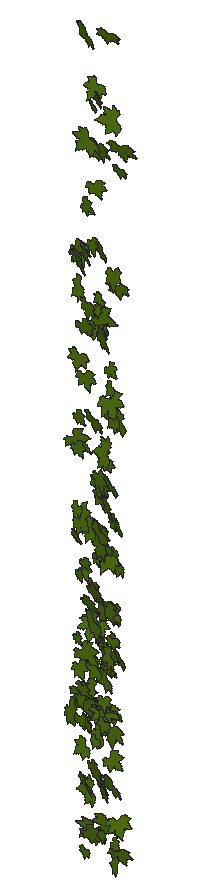
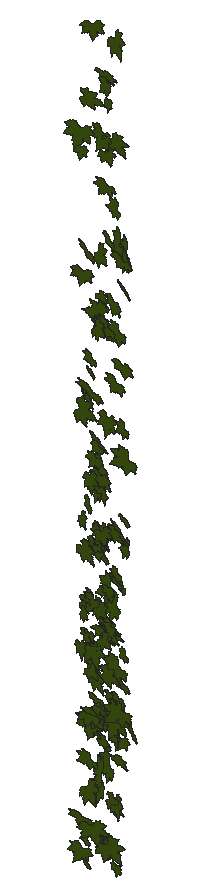
# SketchUp Ruby script. Lengths in inches.
U = 1.inch
M = Sketchup.active_model
def pt(a) = Geom::Point3d.new(a.map { |v| v * U })
def face(e, loops, mat)
  f = e.add_face(loops[0].map { |a| pt(a) })
  loops[1..].each { |l| e.add_face(l.map { |a| pt(a) }).erase! }
  f.material = f.back_material = mat if mat
  f
end
# faces: each face lists its corners as indices into pts; further lists are holes
def faces(e, pts, list, mat = nil) = list.each { |f| face(e, (f[0].is_a?(Array) ? f : [f]).map { |l| l.map { |i| pts[i] } }, mat) }
# xy, xz, yz: faces in a plane at the given z, y or x. An outline is a flat list of corners, or four numbers for a rectangle; further outlines are holes
def ring(l) = l.size == 4 ? [[l[0], l[1]], [l[2], l[1]], [l[2], l[3]], [l[0], l[3]]] : l.each_slice(2).to_a
def flat(e, list, mat, &to3) = list.each { |f| face(e, (f[0].is_a?(Array) ? f : [f]).map { |l| ring(l).map { |u, v| to3.(u, v) } }, mat) }
def xy(e, z, list, mat = nil) = flat(e, list, mat) { |x, y| [x, y, z] }
def xz(e, y, list, mat = nil) = flat(e, list, mat) { |x, z| [x, y, z] }
def yz(e, x, list, mat = nil) = flat(e, list, mat) { |y, z| [x, y, z] }
def lines(e, pts, list) = list.each { |a, b| e.add_line(pt(pts[a]), pt(pts[b])) }
# prism: a flat outline (further loops are holes) pulled along v
def prism(e, loops, v, mat = nil)
  f = face(e, loops, mat); d = Geom::Vector3d.new(v.map { |x| x * U })
  f.pushpull(f.normal.samedirection?(d) ? d.length : -d.length)
end
def box(e, o, s, mat = nil) = prism(e, [[o, [o[0] + s[0], o[1], o[2]], [o[0] + s[0], o[1] + s[1], o[2]], [o[0], o[1] + s[1], o[2]]]], [0, 0, s[2]], mat)
def at(x, y, z, deg = 0) = Geom::Transformation.translation(pt([x, y, z])) * Geom::Transformation.rotation(ORIGIN, Z_AXIS, deg.degrees)
def axes(o, x, y, z) = Geom::Transformation.new([*x, 0, *y, 0, *z, 0, *pt(o).to_a, 1])
def part(name) = M.definitions.add(name)
# library, detail: a bought-in or finely detailed component or shape, given as its bounding box
def library(name, o, s) = part(name).tap { |d| box(d.entities, o, s) }
def detail(e, o, s) = box(e.add_group.entities, o, s)
def put(e, d, t, mat = nil) = e.add_instance(d, t).tap { |i| i.material = mat if mat }
def group(e, t, mat = nil) = e.add_group.tap { |g| g.transformation = t; g.material = mat if mat }.entities
root = M.entities
M.materials.add("[Vegetation Blur 03]").color = [83, 114, 18]
c1 = part("ivy")
xy(c1.entities,0,[[0.782,0,0.786,0,0.787,0.005,0.789,0.009,0.821,0.072,0.875,0.147,1.001,0.272,1.073,0.331,1.137,0.363,1.178,0.379,1.223,0.384,1.272,0.383,1.311,0.374,1.36,0.355,1.399,0.334,1.491,0.285,1.541,0.244,1.583,0.199,1.617,0.15,1.64,0.128,1.662,0.115,1.717,0.105,1.745,0.093,1.784,0.054,1.819,0.057,1.854,0.064,1.882,0.075,1.896,0.074,1.91,0.071,1.937,0.063,1.964,0.053,1.99,0.038,2.016,0.015,2.034,0.002,2.04,0,2.038,0.003,2.036,0.007,2.033,0.038,2.036,0.068,2.045,0.1,2.055,0.116,2.064,0.123,2.077,0.129,2.088,0.129,2.106,0.132,2.118,0.13,2.179,0.132,2.207,0.133,2.225,0.133,2.242,0.138,2.22,0.162,2.207,0.186,2.206,0.213,2.212,0.236,2.228,0.262,2.247,0.274,2.298,0.283,2.355,0.294,2.37,0.296,2.376,0.295,2.377,0.3,2.377,0.303,2.385,0.329,2.411,0.37,2.426,0.392,2.449,0.407,2.511,0.426,2.561,0.444,2.619,0.466,2.589,0.469,2.561,0.476,2.501,0.5,2.449,0.516,2.424,0.523,2.401,0.535,2.377,0.556,2.372,0.568,2.36,0.575,2.268,0.586,2.225,0.592,2.207,0.599,2.194,0.61,2.143,0.65,2.13,0.664,2.122,0.682,2.123,0.7,2.13,0.719,2.148,0.75,2.17,0.781,2.195,0.807,2.221,0.828,2.284,0.874,2.291,0.88,2.288,0.887,2.276,0.9,2.267,0.916,2.265,0.933,2.273,0.967,2.292,1.002,2.313,1.03,2.334,1.054,2.348,1.067,2.358,1.074,2.363,1.076,2.362,1.081,2.35,1.094,2.347,1.11,2.35,1.143,2.359,1.18,2.385,1.254,2.415,1.324,2.448,1.393,2.45,1.4,2.446,1.398,2.44,1.394,2.427,1.383,2.402,1.36,2.376,1.339,2.345,1.324,2.305,1.309,2.282,1.303,2.273,1.306,2.245,1.294,2.212,1.287,2.187,1.291,2.163,1.301,2.142,1.316,2.134,1.327,2.124,1.325,2.09,1.292,2.053,1.259,2.014,1.234,1.973,1.215,1.954,1.21,1.931,1.208,1.909,1.212,1.893,1.22,1.879,1.233,1.872,1.248,1.867,1.281,1.864,1.319,1.821,1.258,1.773,1.197,1.726,1.141,1.698,1.121,1.679,1.116,1.666,1.117,1.647,1.122,1.632,1.129,1.62,1.141,1.617,1.154,1.617,1.219,1.621,1.254,1.623,1.268,1.623,1.281,1.618,1.314,1.606,1.346,1.603,1.375,1.607,1.403,1.603,1.467,1.599,1.499,1.605,1.525,1.614,1.552,1.629,1.577,1.635,1.589,1.629,1.587,1.618,1.582,1.596,1.566,1.581,1.556,1.568,1.552,1.557,1.55,1.545,1.553,1.531,1.562,1.522,1.572,1.504,1.591,1.486,1.611,1.474,1.631,1.457,1.666,1.455,1.684,1.457,1.698,1.452,1.715,1.444,1.728,1.424,1.754,1.419,1.772,1.423,1.786,1.434,1.819,1.444,1.848,1.446,1.855,1.44,1.861,1.43,1.867,1.386,1.904,1.349,1.948,1.326,1.973,1.31,1.995,1.288,2.048,1.284,2.153,1.287,2.254,1.284,2.255,1.282,2.253,1.278,2.247,1.274,2.237,1.266,2.216,1.226,2.125,1.208,2.076,1.184,2.033,1.155,1.984,1.135,1.942,1.111,1.899,1.083,1.861,1.053,1.85,1.059,1.83,1.061,1.809,1.056,1.79,1.049,1.767,1.04,1.749,1.018,1.733,0.994,1.726,0.942,1.734,0.95,1.6875,0.944,1.645,0.932,1.608,0.911,1.585,0.881,1.58,0.854,1.582,0.828,1.588,0.785,1.618,0.773,1.625,0.775,1.614,0.779,1.598,0.796,1.502,0.818,1.402,0.861,1.283,0.882,1.224,0.894,1.174,0.892,1.148,0.886,1.123,0.881,1.107,0.872,1.099,0.849,1.094,0.818,1.092,0.789,1.098,0.762,1.107,0.753,1.113,0.721,1.139,0.698,1.163,0.678,1.194,0.665,1.224,0.628,1.28,0.612,1.312,0.606,1.327,0.606,1.314,0.599,1.282,0.594,1.267,0.581,1.256,0.544,1.245,0.512,1.244,0.473,1.249,0.444,1.256,0.382,1.288,0.339,1.306,0.324,1.316,0.317,1.324,0.309,1.326,0.27,1.314,0.227,1.313,0.185,1.3125,0.152,1.317,0.122,1.328,0.092,1.345,0.073,1.353,0.079,1.338,0.092,1.308,0.117,1.249,0.13,1.215,0.139,1.164,0.147,1.148,0.157,1.136,0.163,1.122,0.174,1.086,0.177,1.067,0.182,1.054,0.186,1.043,0.191,1.038,0.211,1.028,0.237,1.005,0.25,0.974,0.253,0.96,0.25,0.944,0.242,0.914,0.243,0.906,0.249,0.902,0.26,0.894,0.289,0.88,0.307,0.873,0.322,0.862,0.364,0.799,0.403,0.738,0.431,0.709,0.439,0.691,0.441,0.678,0.4375,0.66,0.428,0.645,0.394,0.623,0.303,0.594,0.255,0.581,0.214,0.577,0.179,0.573,0.173,0.568,0.175,0.561,0.167,0.55,0.141,0.523,0.113,0.503,0.077,0.49,0.045,0.486,0.026,0.485,0.019,0.486,0.011,0.483,0,0.471,0.014,0.467,0.044,0.455,0.058,0.447,0.07,0.438,0.097,0.411,0.125,0.394,0.158,0.377,0.174,0.366,0.182,0.359,0.185,0.361,0.242,0.331,0.253,0.316,0.258,0.303,0.262,0.283,0.274,0.278,0.308,0.274,0.341,0.252,0.366,0.226,0.366,0.222,0.37,0.22,0.38,0.221,0.395,0.221,0.425,0.216,0.45,0.207,0.465,0.192,0.473,0.178,0.484,0.15,0.489,0.116,0.483,0.089,0.468,0.058,0.45,0.035,0.435,0.018,0.429,0.011,0.434,0.012,0.438,0.014,0.469,0.019,0.542,0.016,0.581,0.015,0.612,0.027,0.68,0.055,0.696,0.057,0.712,0.052,0.73,0.045,0.741,0.036,0.766,0.014]])
put(root,c1,axes([74.63,173.7,60.75],[0.26152,-0.04302,0.44662],[0.5117,-0.42542,-0.20602],[-0.19512,-1.17335,0.05832]),"[Vegetation Blur 03]")
put(root,c1,axes([74.51,173.7,74.86],[0.3615,0.01419,0.44771],[0.54841,0.02846,-0.29509],[0.01534,-1.35164,-0.00151]),"[Vegetation Blur 03]")
put(root,c1,axes([75.65,173.7,97.39],[0.37946,-0.0754,-0.40939],[-0.47883,0.34147,-0.30552],[-0.15388,-1.24846,-0.05884]),"[Vegetation Blur 03]")
put(root,c1,axes([75.28,173.7,72.12],[0.34373,-0.18323,-0.04475],[-0.06771,-0.09451,-0.28552],[-0.07969,-0.71,0.04955]),"[Vegetation Blur 03]")
put(root,c1,axes([75.15,173.7,64.84],[0.19414,-0.08015,0.20136],[0.24242,-0.09451,-0.1616],[-0.0602,-0.6391,-0.00136]),"[Vegetation Blur 03]")
put(root,c1,axes([75.01,173.7,80.1],[0.54066,-0.11979,-0.01485],[-0.02304,-0.09186,-0.44216],[-0.05647,-1.10941,0.03821]),"[Vegetation Blur 03]")
put(root,c1,axes([74.99,173.7,74.84],[0.30004,-0.03578,0.23182],[0.28092,-0.09842,-0.24458],[-0.04545,-0.84451,0.01868]),"[Vegetation Blur 03]")
put(root,c1,axes([75.03,173.7,60.78],[0.44477,-0.01678,0.0841],[0.10333,0.04659,-0.36253],[-0.00282,-0.93833,-0.0195]),"[Vegetation Blur 03]")
put(root,c1,axes([75.14,173.7,70.17],[0.15681,-0.19135,0.27864],[0.34217,-0.11382,-0.14055],[-0.09017,-0.7647,-0.0488]),"[Vegetation Blur 03]")
put(root,c1,axes([75.1,173.7,76.4375],[0.23733,-0.08095,0.26556],[0.32364,-0.07275,-0.19614],[-0.05179,-0.82556,-0.00876]),"[Vegetation Blur 03]")
put(root,c1,axes([74.89,173.7,85.21],[0.44354,0.00148,0.25414],[0.30752,-0.17731,-0.35733],[-0.04893,-1.101,0.05789]),"[Vegetation Blur 03]")
put(root,c1,axes([75.64,173.7,57.88],[0.41747,-0.18159,-0.28175],[-0.32214,0.27535,-0.34584],[-0.15229,-1.08022,-0.04079]),"[Vegetation Blur 03]")
put(root,c1,axes([75.3125,173.7,68.32],[0.21446,-0.11197,0.17329],[0.20462,-0.11686,-0.18055],[-0.07858,-0.60992,0.00278]),"[Vegetation Blur 03]")
put(root,c1,axes([74.93,173.7,85.11],[0.28904,-0.06987,0.39444],[0.46239,-0.30604,-0.23421],[-0.14468,-1.11768,0.03947]),"[Vegetation Blur 03]")
put(root,c1,axes([75.56,173.7,84.16],[0.42016,-0.3703,-0.17602],[-0.23818,-0.04638,-0.36333],[-0.14889,-0.97076,0.0845]),"[Vegetation Blur 03]")
put(root,c1,axes([74.8,173.7,61.94],[0.46309,-0.00814,0.32802],[0.3991,0.15897,-0.37467],[0.04767,-1.25175,-0.04972]),"[Vegetation Blur 03]")
put(root,c1,axes([75.05,173.7,63.31],[0.35031,-0.0224,0.27157],[0.32357,-0.21117,-0.28075],[-0.0784,-0.97156,0.05476]),"[Vegetation Blur 03]")
put(root,c1,axes([75.76,173.7,59.9],[0.35443,-0.19304,-0.2419],[-0.30587,-0.0509,-0.29211],[-0.05567,-0.94941,0.06485]),"[Vegetation Blur 03]")
put(root,c1,axes([75.72,173.7,91.99],[0.532,-0.08529,-0.32199],[-0.3962,-0.04622,-0.4341],[-0.01987,-1.36215,0.03489]),"[Vegetation Blur 03]")
put(root,c1,axes([75.07,173.7,70.68],[0.16553,0.17765,0.51158],[0.60894,-0.40708,-0.109],[-0.17196,-1.2705,0.10646]),"[Vegetation Blur 03]")
put(root,c1,axes([75.84,173.7,61.0625],[0.30175,-0.15566,-0.18852],[-0.22184,0.13329,-0.25383],[-0.09933,-0.77056,-0.00582]),"[Vegetation Blur 03]")
put(root,c1,axes([75.36,173.7,61.79],[0.24227,-0.06001,0.24324],[0.27574,-0.26297,-0.19314],[-0.11679,-0.74533,0.04856]),"[Vegetation Blur 03]")
put(root,c1,axes([76.33,173.7,57.9],[0.23881,-0.20013,-0.4704],[-0.57401,0.16163,-0.20491],[-0.11037,-1.27363,0.04791]),"[Vegetation Blur 03]")
put(root,c1,axes([75.59,173.7,54.07],[0.31854,-0.11206,-0.01065],[-0.01233,0.01101,-0.26373],[-0.05462,-0.65595,-0.00261]),"[Vegetation Blur 03]")
put(root,c1,axes([75.03,173.7,61.81],[0.67064,-0.03297,0.06761],[0.08405,0.14038,-0.54453],[-0.00745,-1.38343,-0.05687]),"[Vegetation Blur 03]")
put(root,c1,axes([75.37,173.7,62.65],[0.43055,-0.17357,0.04955],[0.0586,-0.03425,-0.35804],[-0.08583,-0.8941,0.0041]),"[Vegetation Blur 03]")
put(root,c1,axes([75.95,173.7,55.68],[0.46314,0.05825,-0.39602],[-0.48604,0.04033,-0.37767],[0.00535,-1.37976,-0.02776]),"[Vegetation Blur 03]")
put(root,c1,axes([75.51,173.7,68.93],[0.24085,-0.07286,0.19486],[0.23769,-0.04913,-0.19858],[-0.04198,-0.69616,-0.00638]),"[Vegetation Blur 03]")
put(root,c1,axes([76.24,173.7,71.6875],[0.31165,-0.23246,-0.38206],[-0.4746,0.04633,-0.26229],[-0.08166,-1.15634,0.0663]),"[Vegetation Blur 03]")
put(root,c1,axes([75.19,173.7,81.35],[0.40049,-0.10291,0.28569],[0.35224,0.02026,-0.32774],[-0.03114,-1.09438,-0.03293]),"[Vegetation Blur 03]")
put(root,c1,axes([76.46,173.7,66.65],[0.20411,-0.06117,-0.44075],[-0.53473,0.15542,-0.16833],[-0.08116,-1.17781,0.00068]),"[Vegetation Blur 03]")
put(root,c1,axes([75.49,173.7,68.47],[0.2517,0.01272,0.24338],[0.28699,-0.2291,-0.19581],[-0.08127,-0.76965,0.06231]),"[Vegetation Blur 03]")
put(root,c1,axes([75.07,173.7,85.12],[0.43009,-0.41994,0.38446],[0.46829,-0.19735,-0.38284],[-0.21039,-1.29771,-0.06619]),"[Vegetation Blur 03]")
put(root,c1,axes([75.28,173.7,78.8],[0.46612,-0.06322,0.21313],[0.25778,-0.10592,-0.38046],[-0.05188,-1.09436,0.02451]),"[Vegetation Blur 03]")
put(root,c1,axes([75.07,173.7,63.9375],[0.4004,-0.01607,0.44585],[0.54595,-0.04146,-0.32681],[-0.02086,-1.39316,0.00458]),"[Vegetation Blur 03]")
put(root,c1,axes([76.54,173.7,63.05],[0.07522,-0.13511,-0.31021],[-0.37954,0.11629,-0.06927],[-0.06884,-0.78881,0.04292]),"[Vegetation Blur 03]")
put(root,c1,axes([76.7,173.7,64.33],[0.13923,-0.07198,-0.4584],[-0.56199,0.04465,-0.11479],[-0.02951,-1.18996,0.02342]),"[Vegetation Blur 03]")
put(root,c1,axes([76.11,173.7,91.09],[0.32097,0.04197,-0.19874],[-0.24426,0.07998,-0.2601],[-0.00735,-0.82521,-0.03532]),"[Vegetation Blur 03]")
put(root,c1,axes([75.63,173.7,87.48],[0.11949,-0.05949,0.35767],[0.43416,-0.12523,-0.09989],[-0.06637,-0.92633,-0.00946]),"[Vegetation Blur 03]")
put(root,c1,axes([76.5,173.7,66.05],[0.16976,0.07158,-0.29867],[-0.3654,0.12339,-0.13369],[-0.04012,-0.82092,-0.04613]),"[Vegetation Blur 03]")
put(root,c1,axes([75.63,173.7,82.96],[0.51145,-0.25079,0.06105],[0.06998,-0.0596,-0.42899],[-0.12471,-1.06199,0.00966]),"[Vegetation Blur 03]")
put(root,c1,axes([76.14,173.7,93.46],[0.26677,-0.13263,-0.08131],[-0.08808,0.11667,-0.22242],[-0.07951,-0.57427,-0.02641]),"[Vegetation Blur 03]")
put(root,c1,axes([75.46,173.7,85.63],[0.38011,-0.35457,0.334],[0.40396,-0.18413,-0.33696],[-0.18436,-1.13452,-0.04969]),"[Vegetation Blur 03]")
put(root,c1,axes([76.02,173.7,68.28],[0.33233,-0.0945,-0.02615],[-0.02986,0.03657,-0.27359],[-0.04737,-0.68607,-0.01098]),"[Vegetation Blur 03]")
put(root,c1,axes([76.74,173.7,86.07],[0.15729,0.04975,-0.38701],[-0.46067,0.26502,-0.11935],[-0.11503,-0.99334,-0.05122]),"[Vegetation Blur 03]")
put(root,c1,axes([76.05,173.7,66.71],[0.56265,-0.26157,-0.25412],[-0.30853,0.09554,-0.47049],[-0.13384,-1.31983,0.01631]),"[Vegetation Blur 03]")
put(root,c1,axes([76.25,173.7,71.48],[0.35115,0.05857,-0.18722],[-0.23024,0.1649,-0.27952],[-0.02054,-0.84722,-0.06735]),"[Vegetation Blur 03]")
put(root,c1,axes([75.61,173.7,54.55],[0.26007,-0.08689,0.38147],[0.46915,0.07766,-0.21026],[0.0126,-1.09796,-0.04506]),"[Vegetation Blur 03]")
put(root,c1,axes([75.72,173.7,66.27],[0.61939,0.05734,-0.0417],[-0.04546,-0.22498,-0.49845],[0.03634,-1.25897,0.08717]),"[Vegetation Blur 03]")
put(root,c1,axes([75.86,173.7,65.87],[0.12985,0.03067,0.35023],[0.42444,-0.14892,-0.10276],[-0.06505,-0.91052,0.02861]),"[Vegetation Blur 03]")
put(root,c1,axes([76.66,173.7,67.54],[0.17674,0.08976,-0.26223],[-0.3229,0.11764,-0.13863],[-0.02967,-0.7454,-0.05345]),"[Vegetation Blur 03]")
put(root,c1,axes([75.85,173.7,77.13],[0.58072,-0.2362,-0.06513],[-0.0644,0.17074,-0.47989],[-0.12408,-1.1941,-0.05574]),"[Vegetation Blur 03]")
put(root,c1,axes([75.61,173.7,66.92],[0.32867,-0.28906,0.36046],[0.45664,0.0115,-0.27589],[-0.07923,-1.13284,-0.09478]),"[Vegetation Blur 03]")
put(root,c1,axes([76.9375,173.7,82.0625],[0.08767,0.08949,-0.34433],[-0.41588,0.19217,-0.06267],[-0.08326,-0.86566,-0.04951]),"[Vegetation Blur 03]")
put(root,c1,axes([76.58,173.7,66.08],[0.25432,-0.19046,-0.24423],[-0.28944,0.16036,-0.22043],[-0.11975,-0.79207,0.0141]),"[Vegetation Blur 03]")
put(root,c1,axes([75.82,173.7,88.9],[0.40459,0.02303,0.19859],[0.2435,-0.01333,-0.3302],[0.00625,-0.97145,0.00924]),"[Vegetation Blur 03]")
put(root,c1,axes([75.96,173.7,85.91],[0.28926,-0.09005,0.2261],[0.2622,-0.20395,-0.23621],[-0.09958,-0.79857,0.03483]),"[Vegetation Blur 03]")
put(root,c1,axes([77.01,173.7,60.75],[0.10121,-0.15146,-0.36108],[-0.44341,0.10659,-0.08981],[-0.06746,-0.92784,0.04863]),"[Vegetation Blur 03]")
put(root,c1,axes([76.34,173.7,60.16],[0.30014,-0.14068,-0.03498],[-0.05049,-0.06238,-0.24906],[-0.06295,-0.62077,0.03295]),"[Vegetation Blur 03]")
put(root,c1,axes([76.72,173.7,83.5],[0.20022,-0.05357,-0.19807],[-0.24233,0.03356,-0.1646],[-0.02917,-0.64656,0.00787]),"[Vegetation Blur 03]")
put(root,c1,axes([77.03,173.7,62.2],[0.11196,0.05174,-0.31654],[-0.38834,-0.01941,-0.09199],[0.01605,-0.83049,-0.01757]),"[Vegetation Blur 03]")
put(root,c1,axes([76.24,173.7,94.85],[0.51677,-0.16,-0.11108],[-0.14975,-0.2188,-0.41446],[-0.04632,-1.0777,0.10064]),"[Vegetation Blur 03]")
put(root,c1,axes([75.79,173.7,81.24],[0.28098,0.0713,0.44477],[0.5442,-0.14112,-0.22543],[-0.04527,-1.25382,0.05067]),"[Vegetation Blur 03]")
put(root,c1,axes([76.28,173.7,82.61],[0.25172,-0.04798,0.1294],[0.15152,-0.12662,-0.20371],[-0.0522,-0.59895,0.0327]),"[Vegetation Blur 03]")
put(root,c1,axes([76.38,173.7,71.53],[0.559,-0.25408,-0.226],[-0.26774,0.14716,-0.46713],[-0.14227,-1.27524,-0.00888]),"[Vegetation Blur 03]")
put(root,c1,axes([76.29,173.7,69.52],[0.23635,-0.06465,0.19523],[0.22776,-0.16748,-0.19239],[-0.07957,-0.67142,0.02919]),"[Vegetation Blur 03]")
put(root,c1,axes([76.5625,173.7,73.35],[0.41365,-0.19736,-0.16762],[-0.20533,0.04633,-0.34609],[-0.09602,-0.94924,0.01796]),"[Vegetation Blur 03]")
put(root,c1,axes([76.12,173.7,94.01],[0.40968,-0.27629,0.16507],[0.21084,0.00024,-0.34848],[-0.12034,-0.94019,-0.0486]),"[Vegetation Blur 03]")
put(root,c1,axes([76.32,173.7,60.81],[0.09158,0.04301,0.34718],[0.42504,-0.06647,-0.07338],[-0.02723,-0.89296,0.02219]),"[Vegetation Blur 03]")
put(root,c1,axes([76.97,173.7,63.93],[0.35185,-0.14327,-0.37157],[-0.44566,0.19161,-0.29272],[-0.11623,-1.16844,-0.00244]),"[Vegetation Blur 03]")
put(root,c1,axes([75.94,173.7,67.6875],[0.38346,-0.30784,0.36497],[0.45646,-0.05536,-0.32679],[-0.11835,-1.21097,-0.07784]),"[Vegetation Blur 03]")
put(root,c1,axes([76.22,173.7,73.91],[0.59559,-0.20487,-0.02237],[-0.02751,0.00349,-0.49282],[-0.09953,-1.2269,0.00233]),"[Vegetation Blur 03]")
put(root,c1,axes([76.83,173.7,62.13],[0.45581,0.11699,-0.31525],[-0.38742,-0.0162,-0.37405],[0.04848,-1.22937,-0.02507]),"[Vegetation Blur 03]")
put(root,c1,axes([76.08,173.7,91.49],[0.6079,-0.24736,0.08777],[0.11732,0.08596,-0.50313],[-0.11068,-1.26744,-0.05125]),"[Vegetation Blur 03]")
put(root,c1,axes([76.41,173.7,70.82],[0.56324,-0.31646,-0.09717],[-0.11977,0.02711,-0.47626],[-0.15324,-1.18433,0.01506]),"[Vegetation Blur 03]")
put(root,c1,axes([76.47,173.7,65.51],[0.3306,-0.20851,0.08999],[0.10594,-0.063,-0.2822],[-0.10584,-0.71438,-0.00138]),"[Vegetation Blur 03]")
put(root,c1,axes([75.96,173.7,58.5],[0.44878,-0.3413,0.36007],[0.4395,-0.14984,-0.38721],[-0.17027,-1.28634,-0.05043]),"[Vegetation Blur 03]")
put(root,c1,axes([76.72,173.7,65.4],[0.54219,-0.07189,-0.27942],[-0.3337,0.21166,-0.43986],[-0.08416,-1.30245,-0.05606]),"[Vegetation Blur 03]")
put(root,c1,axes([76.59,173.7,97.41],[0.46012,0.08661,-0.09796],[-0.12471,0.12465,-0.37281],[0.02504,-0.97055,-0.05662]),"[Vegetation Blur 03]")
put(root,c1,axes([76.5625,173.7,56.16],[0.58678,0.063,-0.19417],[-0.23912,0.05083,-0.47872],[0.01906,-1.30195,-0.02809]),"[Vegetation Blur 03]")
put(root,c1,axes([76.51,173.7,55.27],[0.34382,-0.15266,0.07768],[0.0934,-0.03785,-0.28706],[-0.07642,-0.73315,-0.00136]),"[Vegetation Blur 03]")
put(root,c1,axes([76.07,173.7,61.53],[0.59488,0.11123,0.16598],[0.20655,-0.0688,-0.48585],[0.04022,-1.29188,0.04016]),"[Vegetation Blur 03]")
put(root,c1,axes([76.54,173.7,58.05],[0.51362,-0.33546,-0.11294],[-0.11227,0.20752,-0.43703],[-0.18199,-1.07476,-0.04914]),"[Vegetation Blur 03]")
put(root,c1,axes([77.11,173.7,64.17],[0.24584,0.04332,-0.24097],[-0.29547,0.08344,-0.19842],[-0.01781,-0.78621,-0.03434]),"[Vegetation Blur 03]")
put(root,c1,axes([77.45,173.7,76.09],[0.21833,-0.37386,-0.44692],[-0.55988,0.15366,-0.2024],[-0.13932,-1.20335,0.113]),"[Vegetation Blur 03]")
put(root,c1,axes([77.2,173.7,58.26],[0.33588,0.02262,-0.39753],[-0.47681,0.26549,-0.26596],[-0.10014,-1.18823,-0.067]),"[Vegetation Blur 03]")
put(root,c1,axes([76.25,173.7,81.59],[0.09221,0.01276,0.54145],[0.66339,-0.02223,-0.07517],[-0.00985,-1.37816,0.00623]),"[Vegetation Blur 03]")
put(root,c1,axes([76.54,173.7,75.17],[0.25,-0.03131,0.17773],[0.21716,-0.03407,-0.2044],[-0.02234,-0.68141,0.00205]),"[Vegetation Blur 03]")
put(root,c1,axes([76.51,173.7,66.53],[0.13511,-0.04438,0.35866],[0.42367,-0.24214,-0.11102],[-0.11873,-0.91459,0.01199]),"[Vegetation Blur 03]")
put(root,c1,axes([76.75,173.7,61.24],[0.37736,-0.14693,-0.03133],[-0.04655,-0.08489,-0.31089],[-0.06637,-0.77592,0.03994]),"[Vegetation Blur 03]")
put(root,c1,axes([76.58,173.7,62.22],[0.36114,-0.04689,0.10699],[0.12628,-0.12494,-0.29255],[-0.0419,-0.78067,0.04039]),"[Vegetation Blur 03]")
put(root,c1,axes([76.98,173.7,64.5625],[0.39633,-0.13888,-0.234],[-0.27566,0.17367,-0.32719],[-0.1038,-0.99151,-0.02453]),"[Vegetation Blur 03]")
put(root,c1,axes([76.73,173.7,70.66],[0.10493,-0.03643,0.24088],[0.29195,-0.08918,-0.08683],[-0.04677,-0.63839,-0.00162]),"[Vegetation Blur 03]")
put(root,c1,axes([76.5625,173.7,74.63],[0.3534,-0.02851,0.14206],[0.17452,0.03242,-0.28817],[-0.00545,-0.81,-0.01653]),"[Vegetation Blur 03]")
put(root,c1,axes([76.7,173.7,70.42],[0.40755,-0.11351,-0.00014],[0.00098,0.01751,-0.33557],[-0.05515,-0.83847,-0.00699]),"[Vegetation Blur 03]")
put(root,c1,axes([77.01,173.7,74.03],[0.4235,-0.13743,-0.21645],[-0.24668,0.24247,-0.3457],[-0.1181,-0.99928,-0.05411]),"[Vegetation Blur 03]")
put(root,c1,axes([76.78,173.7,63.86],[0.26031,-0.0805,0.12545],[0.1556,0.01165,-0.21388],[-0.03078,-0.62197,-0.02024]),"[Vegetation Blur 03]")
put(root,c1,axes([76.26,173.7,73.87],[0.47957,-0.26061,0.31785],[0.37221,-0.23733,-0.40467],[-0.1708,-1.24893,0.01057]),"[Vegetation Blur 03]")
put(root,c1,axes([76.65,173.7,67.28],[0.41549,-0.08208,0.11963],[0.15106,0.12998,-0.33542],[-0.01613,-0.89729,-0.05953]),"[Vegetation Blur 03]")
put(root,c1,axes([77.3125,173.7,65.2],[0.33509,-0.2609,-0.26753],[-0.3303,0.08476,-0.28857],[-0.12012,-0.96089,0.04719]),"[Vegetation Blur 03]")
put(root,c1,axes([77.64,173.7,65.78],[0.07952,-0.02515,-0.25316],[-0.29832,0.17612,-0.06516],[-0.08589,-0.63499,-0.00805]),"[Vegetation Blur 03]")
put(root,c1,axes([76.76,173.7,70.26],[0.59751,-0.1415,-0.08723],[-0.11552,-0.16395,-0.48523],[-0.05298,-1.23827,0.07421]),"[Vegetation Blur 03]")
put(root,c1,axes([77.88,173.7,93.66],[0.17867,-0.14742,-0.47769],[-0.58909,-0.10072,-0.14187],[0.02629,-1.25528,0.06748]),"[Vegetation Blur 03]")
put(root,c1,axes([78.06,173.7,77.72],[0.10377,0.02186,-0.53621],[-0.65451,0.12482,-0.08356],[-0.05827,-1.36305,-0.01625]),"[Vegetation Blur 03]")
put(root,c1,axes([76.53,173.7,81.17],[0.29678,-0.27186,0.42657],[0.50911,-0.26247,-0.26224],[-0.17731,-1.20867,-0.039]),"[Vegetation Blur 03]")
put(root,c1,axes([77.85,173.7,66.94],[0.04974,-0.00028,-0.27725],[-0.32677,0.19308,-0.03908],[-0.09286,-0.67961,-0.01099]),"[Vegetation Blur 03]")
put(root,c1,axes([77.9375,173.7,67.46],[0.08632,-0.07212,-0.36138],[-0.4424,0.06914,-0.07256],[-0.03977,-0.92577,0.02273]),"[Vegetation Blur 03]")
put(root,c1,axes([76.82,173.7,57.62],[0.09448,-0.24372,0.47773],[0.55916,-0.39227,-0.10514],[-0.20978,-1.15536,-0.06508]),"[Vegetation Blur 03]")
put(root,c1,axes([77.62,173.7,70.4375],[0.39881,-0.16855,-0.40776],[-0.49292,0.16963,-0.33214],[-0.11562,-1.30452,0.00949]),"[Vegetation Blur 03]")
put(root,c1,axes([76.95,173.7,79.48],[0.21376,-0.00368,0.2636],[0.3197,-0.11113,-0.17293],[-0.04601,-0.78924,0.02312]),"[Vegetation Blur 03]")
put(root,c1,axes([77.32,173.7,79.12],[0.30532,-0.22387,-0.07925],[-0.10993,-0.04866,-0.26046],[-0.09582,-0.65751,0.04626]),"[Vegetation Blur 03]")
put(root,c1,axes([77.85,173.7,54.12],[0.10497,-0.16799,-0.28426],[-0.34085,0.17977,-0.10055],[-0.10859,-0.72666,0.04084]),"[Vegetation Blur 03]")
put(root,c1,axes([77.12,173.7,65.5625],[0.3425,-0.04443,0.04433],[0.05384,-0.01893,-0.28004],[-0.02276,-0.71335,0.00467]),"[Vegetation Blur 03]")
put(root,c1,axes([76.69,173.7,61.03],[0.66487,-0.12258,0.05657],[0.06821,-0.03171,-0.54475],[-0.06083,-1.37523,0.00752]),"[Vegetation Blur 03]")
put(root,c1,axes([77.74,173.7,71.85],[0.19183,-0.05588,-0.2698],[-0.31224,0.23474,-0.15552],[-0.11192,-0.75067,-0.02855]),"[Vegetation Blur 03]")
put(root,c1,axes([76.74,173.7,66.98],[0.40007,-0.13518,0.27607],[0.33165,-0.13835,-0.33079],[-0.0935,-1.06919,0.0079]),"[Vegetation Blur 03]")
put(root,c1,axes([76.82,173.7,58.75],[0.24435,0.09355,0.35761],[0.44053,-0.04867,-0.19849],[0.00137,-1.03125,0.04181]),"[Vegetation Blur 03]")
put(root,c1,axes([76.52,173.7,77.74],[0.49312,0.07516,0.37451],[0.45503,-0.28887,-0.38996],[-0.06962,-1.3557,0.10386]),"[Vegetation Blur 03]")
put(root,c1,axes([76.68,173.7,72.64],[0.40386,-0.35784,0.38449],[0.46593,-0.19708,-0.35483],[-0.18733,-1.26162,-0.05362]),"[Vegetation Blur 03]")
put(root,c1,axes([77.34,173.7,54.54],[0.09713,0.02395,0.23937],[0.28996,-0.10667,-0.07669],[-0.04564,-0.62678,0.0222]),"[Vegetation Blur 03]")
put(root,c1,axes([77.15,173.7,84.24],[0.48068,0.01776,0.03152],[0.03794,0.06838,-0.39147],[0.01124,-0.98997,-0.02647]),"[Vegetation Blur 03]")
put(root,c1,axes([77.55,173.7,77.92],[0.4464,-0.35085,-0.18371],[-0.23796,-0.0009,-0.38487],[-0.15203,-1.02878,0.06299]),"[Vegetation Blur 03]")
put(root,c1,axes([77.26,173.7,71.75],[0.21308,-0.12887,0.25392],[0.29486,-0.2048,-0.18116],[-0.11737,-0.74847,0.00585]),"[Vegetation Blur 03]")
put(root,c1,axes([77.13,173.7,54.32],[0.46585,0.02288,0.14137],[0.17091,0.11775,-0.37813],[0.0303,-1.01595,-0.04064]),"[Vegetation Blur 03]")
put(root,c1,axes([77.68,173.7,65.05],[0.36602,-0.17334,-0.17958],[-0.2031,0.19186,-0.30487],[-0.11941,-0.85763,-0.0319]),"[Vegetation Blur 03]")
put(root,c1,axes([77.08,173.7,91.67],[0.63593,0.00439,0.02808],[0.0337,0.19557,-0.51321],[0.00724,-1.29586,-0.07736]),"[Vegetation Blur 03]")
put(root,c1,axes([77.51,173.7,90.55],[0.37054,-0.08411,-0.02834],[-0.02969,0.09383,-0.30232],[-0.04467,-0.76008,-0.03419]),"[Vegetation Blur 03]")
put(root,c1,axes([77.06,173.7,55.84],[0.46596,0.12424,0.22352],[0.28037,-0.18097,-0.37349],[0.00652,-1.09739,0.0869]),"[Vegetation Blur 03]")
put(root,c1,axes([77.1,173.7,84.9],[0.46976,-0.15316,0.21327],[0.23871,-0.28032,-0.3819],[-0.12977,-1.07007,0.06952]),"[Vegetation Blur 03]")
